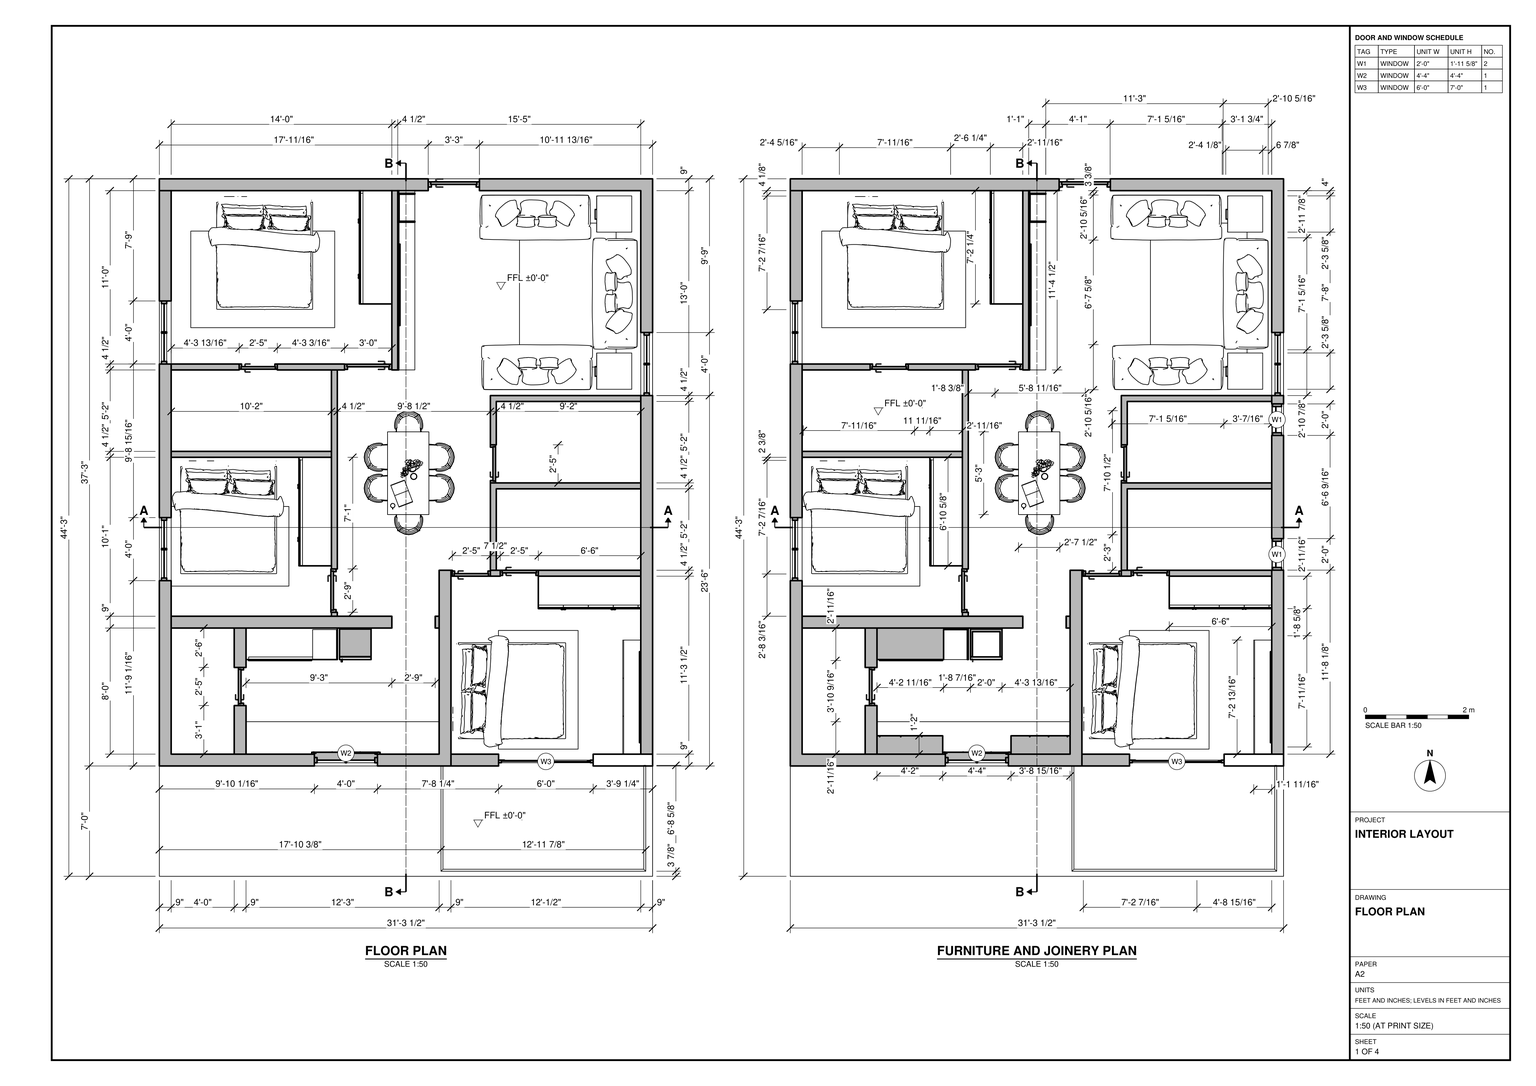
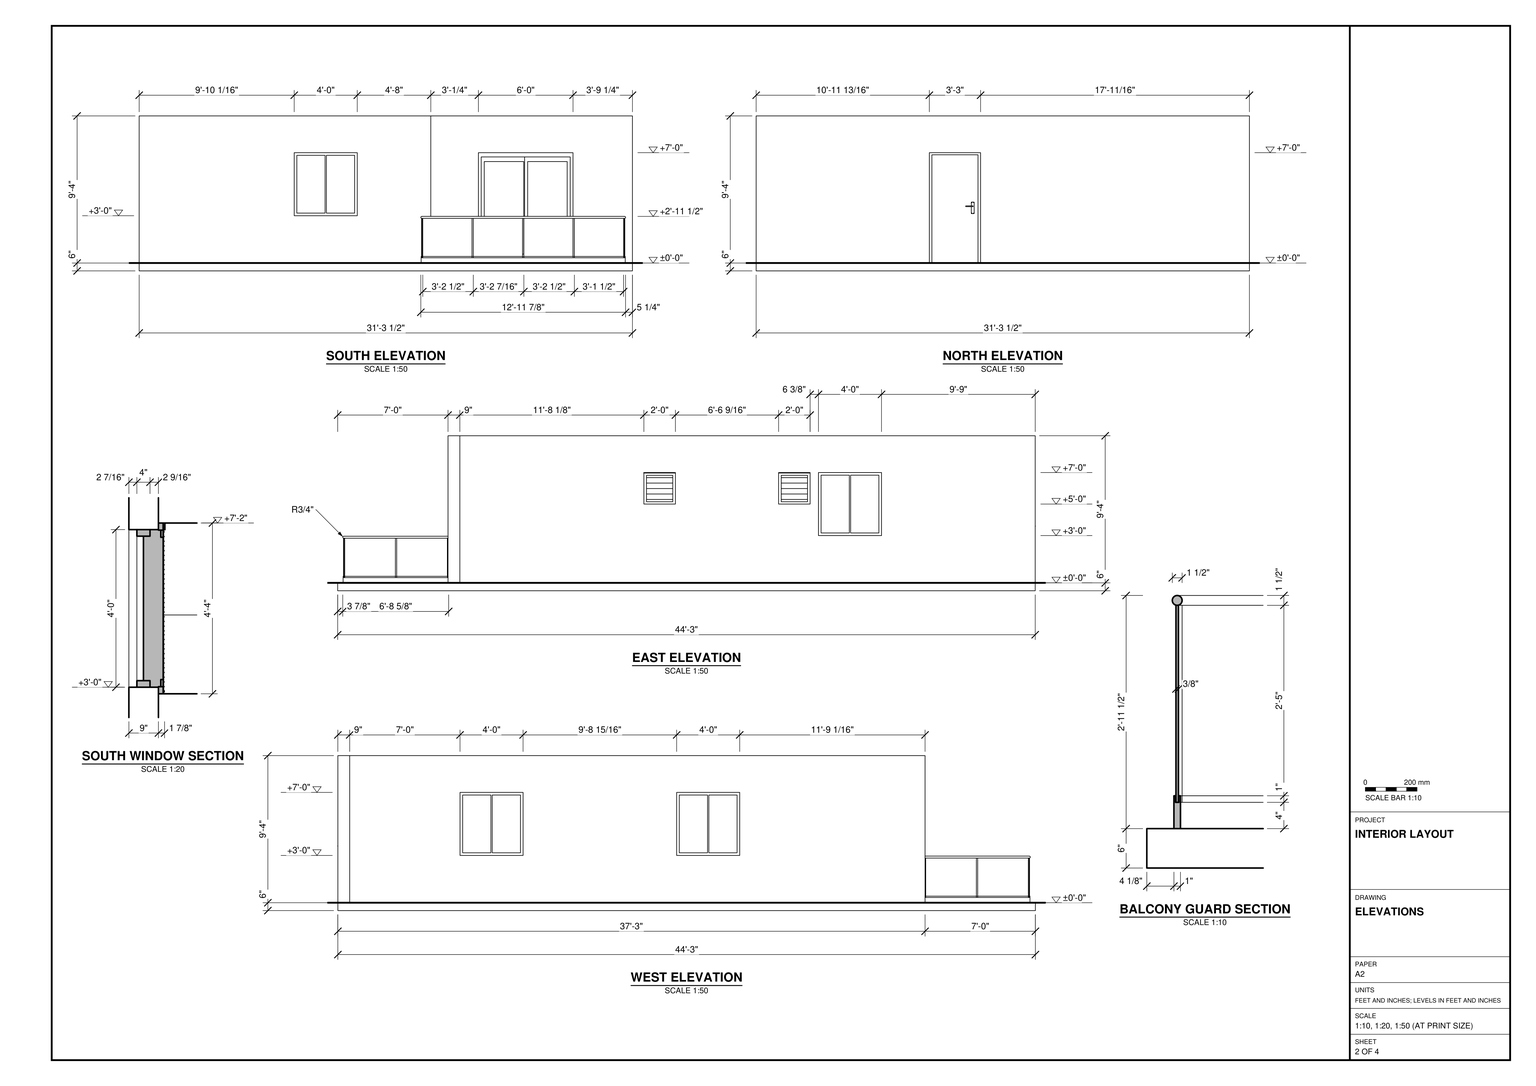
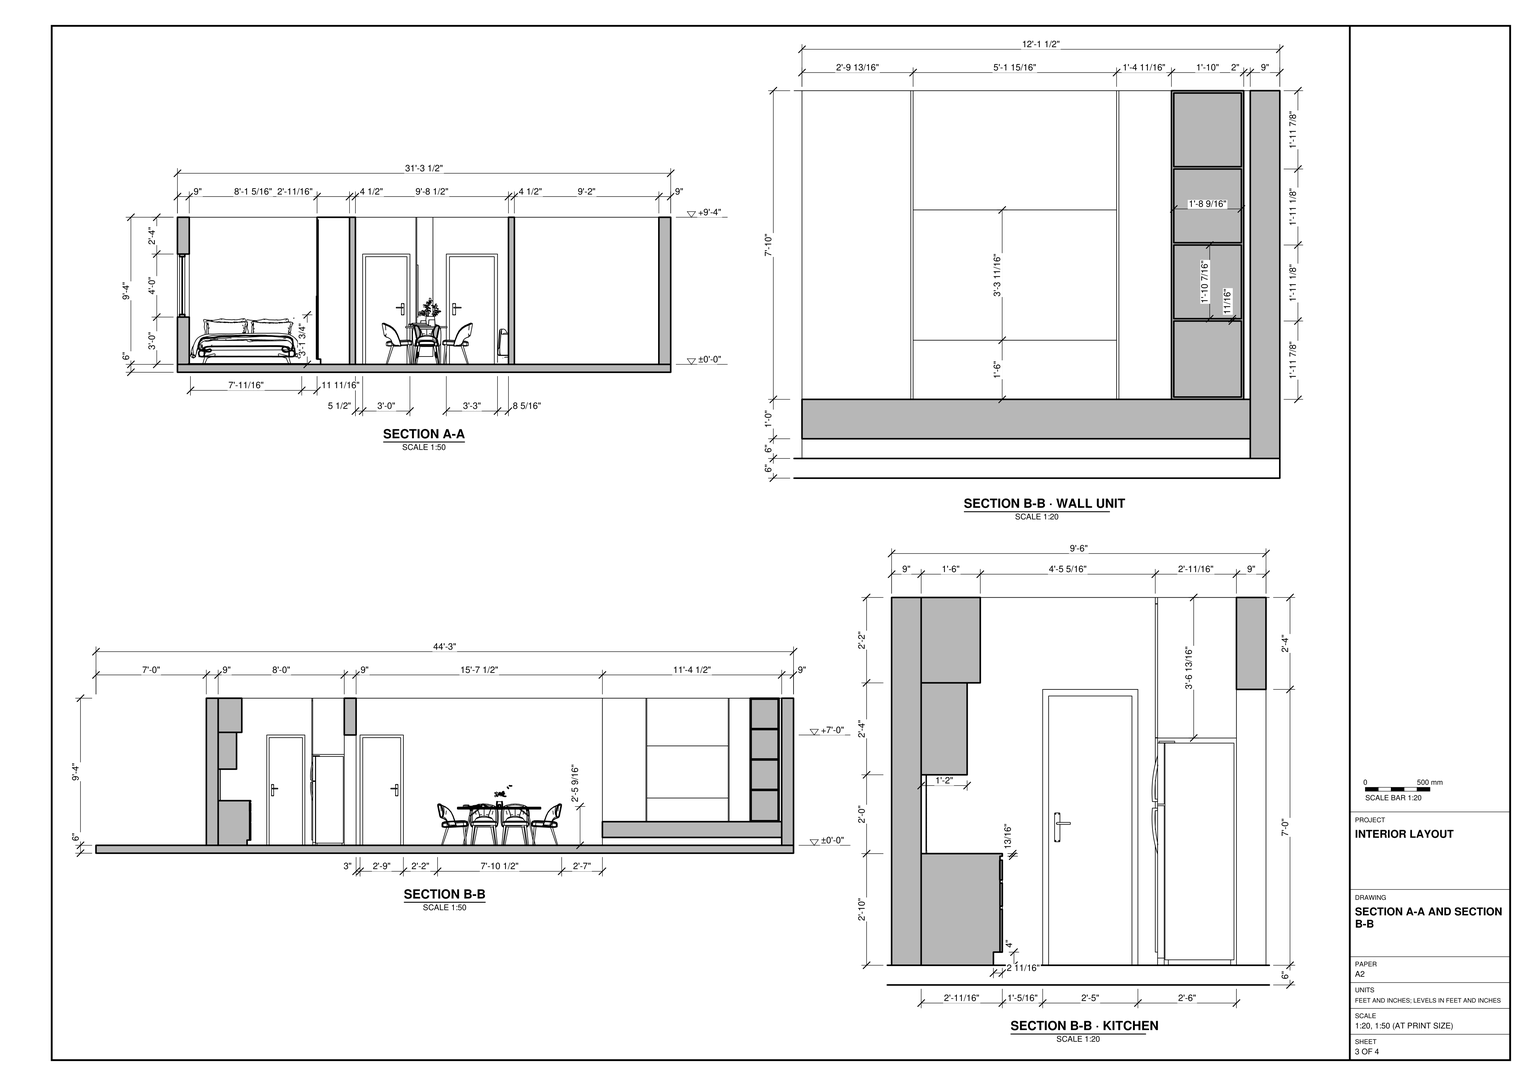
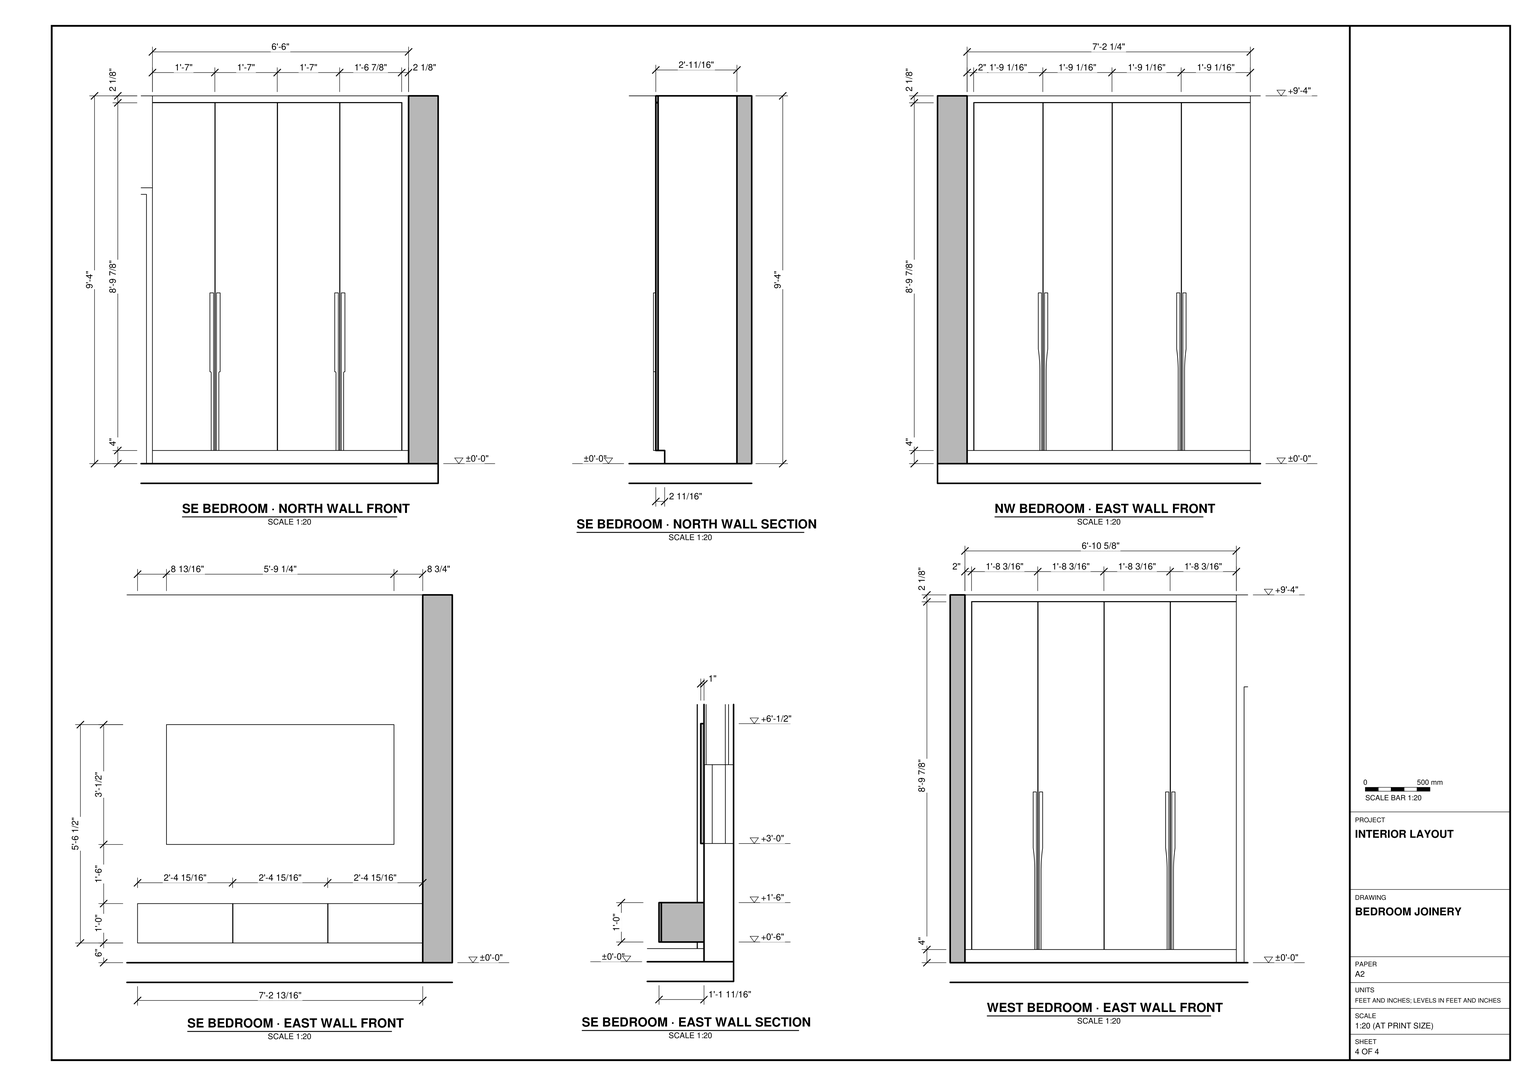
Build the single-storey interior in SketchUp using task_files/diagram_01.pdf. Work in feet and inches. Set the finished floor at ±0'-0". The overall model, including the balcony, is 31'-3 1/2" east to west, 44'-3 1/8" north to south and 9'-10" high.

Model the 6" floor slab and raise the walls 9'-4" above the finished floor. Follow the drawn wall thicknesses, distinguishing the 9" perimeter walls from the lighter 4 1/2" partitions. Lay out the bedrooms on the west side and at the southeast corner, the living area at the northeast, the central dining area and the kitchen at the southwest. Preserve the smaller enclosed rooms and the doorways connecting the spaces. Fit the doors, window units and high east-wall ventilators to the openings shown in plan and elevation. Extend the balcony outside the southeast bedroom and model its panelled glass guard using the guard section.

Use the furniture plan to size and orient the beds, bedroom storage, sofas, side tables, dining table and chairs. Use the sections to build the living-area wall unit with its low base and shelving, and the kitchen with its worktop, cabinets and refrigerator. Decor and loose items, including rugs, cushions and appliances, may be any suitable library components.

Keep the shell elements and each furniture or joinery piece in separate groups or components, and use components for repeated parts. Save one SketchUp model as output_files/furnished_three_bedroom_interior_with_a_south_balcony.skp.

# SketchUp Ruby script. Lengths in inches.
U = 1.inch
M = Sketchup.active_model
def pt(a) = Geom::Point3d.new(a.map { |v| v * U })
def face(e, loops, mat)
  f = e.add_face(loops[0].map { |a| pt(a) })
  loops[1..].each { |l| e.add_face(l.map { |a| pt(a) }).erase! }
  f.material = f.back_material = mat if mat
  f
end
# faces: each face lists its corners as indices into pts; further lists are holes
def faces(e, pts, list, mat = nil) = list.each { |f| face(e, (f[0].is_a?(Array) ? f : [f]).map { |l| l.map { |i| pts[i] } }, mat) }
# xy, xz, yz: faces in a plane at the given z, y or x. An outline is a flat list of corners, or four numbers for a rectangle; further outlines are holes
def ring(l) = l.size == 4 ? [[l[0], l[1]], [l[2], l[1]], [l[2], l[3]], [l[0], l[3]]] : l.each_slice(2).to_a
def flat(e, list, mat, &to3) = list.each { |f| face(e, (f[0].is_a?(Array) ? f : [f]).map { |l| ring(l).map { |u, v| to3.(u, v) } }, mat) }
def xy(e, z, list, mat = nil) = flat(e, list, mat) { |x, y| [x, y, z] }
def xz(e, y, list, mat = nil) = flat(e, list, mat) { |x, z| [x, y, z] }
def yz(e, x, list, mat = nil) = flat(e, list, mat) { |y, z| [x, y, z] }
def lines(e, pts, list) = list.each { |a, b| e.add_line(pt(pts[a]), pt(pts[b])) }
# prism: a flat outline (further loops are holes) pulled along v
def prism(e, loops, v, mat = nil)
  f = face(e, loops, mat); d = Geom::Vector3d.new(v.map { |x| x * U })
  f.pushpull(f.normal.samedirection?(d) ? d.length : -d.length)
end
def box(e, o, s, mat = nil) = prism(e, [[o, [o[0] + s[0], o[1], o[2]], [o[0] + s[0], o[1] + s[1], o[2]], [o[0], o[1] + s[1], o[2]]]], [0, 0, s[2]], mat)
def at(x, y, z, deg = 0) = Geom::Transformation.translation(pt([x, y, z])) * Geom::Transformation.rotation(ORIGIN, Z_AXIS, deg.degrees)
def axes(o, x, y, z) = Geom::Transformation.new([*x, 0, *y, 0, *z, 0, *pt(o).to_a, 1])
def part(name) = M.definitions.add(name)
# library, detail: a bought-in or finely detailed component or shape, given as its bounding box
def library(name, o, s) = part(name).tap { |d| box(d.entities, o, s) }
def detail(e, o, s) = box(e.add_group.entities, o, s)
def put(e, d, t, mat = nil) = e.add_instance(d, t).tap { |i| i.material = mat if mat }
def group(e, t, mat = nil) = e.add_group.tap { |g| g.transformation = t; g.material = mat if mat }.entities
root = M.entities
M.materials.add("0516 AP 9704 Lake Supreme-N").color = [0, 147, 150]
M.materials.add("0604 AP 9737 Aquamarine Pop-N").color = [0, 150, 118]
M.materials.add("0607 AP 9740 Bright Teal-N").color = [0, 121, 105]
M.materials.add("0908 AP 7841 CORN FIELD").color = [237, 222, 177]
M.materials.add("0916 AP 7849 PEBBLE MOSS").color = [210, 196, 159]
M.materials.add("0932 AP 7856 GOLDILOCKS").color = [236, 215, 152]
M.materials.add("0944 AP 9875 Lazy Daisy-N").color = [241, 200, 58]
M.materials.add("1160 AP 9961 Cherry Brown-N").color = [109, 68, 67]
M.materials.add("Carpet").color = [165, 157, 133]
M.materials.add("Railing Glass").color = [63, 150, 137]
M.materials["Railing Glass"].alpha = 0.13
M.materials.add("[Color M00]").color = [255, 255, 255]
M.materials.add("[Color M09]").color = [0, 0, 0]
M.materials.add("[Color_002]").color = [198, 198, 198]
M.materials.add("[Translucent Glass Gray]").color = [128, 128, 128]
M.materials["[Translucent Glass Gray]"].alpha = 0.5
M.materials.add("[Translucent Glass Tinted]1").color = [7, 201, 240]
M.materials["[Translucent Glass Tinted]1"].alpha = 0.48
M.materials.add("[Wood Cherry Original]").color = [152, 86, 42]
M.materials.add("[Wood Floor Parquet]").color = [145, 89, 39]
c1 = part("Sliding Window")
xy(c1.entities,0,[[0,0,66.93,1.97]],"[Color M09]")
xy(c1.entities,1.97,[[1.97,0,64.96,0,64.96,0.39,32.7,0.39,32.7,1.18,1.97,1.18],[34.23,1.18,64.96,1.97]],"[Color M09]")
xy(c1.entities,49.21,[[1.97,0,1.97,1.18,32.7,1.18,32.7,0.39,64.96,0.39,64.96,0],[34.23,1.18,64.96,1.97]],"[Color M09]")
xy(c1.entities,51.18,[[0,0,66.93,1.97]],"[Color M09]")
xz(c1.entities,0,[[[0,0,66.93,51.18],[1.97,1.97,64.96,49.21]]],"[Color M09]")
xz(c1.entities,1.18,[[[34.23,1.97,64.96,49.21],[34.85,4.12,62.81,47.07]]],"[Color M09]")
xz(c1.entities,1.97,[[[0,0,66.93,51.18],[1.97,1.97,64.96,49.21]]],"[Color M09]")
yz(c1.entities,0,[[0,0,1.97,51.18]],"[Color M09]")
yz(c1.entities,1.97,[[0,1.97,1.18,49.21]],"[Color M09]")
yz(c1.entities,64.96,[[0,1.97,0.39,49.21],[1.18,1.97,1.97,49.21]],"[Color M09]")
yz(c1.entities,66.93,[[0,0,1.97,51.18]],"[Color M09]")
g1 = group(c1.entities,at(1.97,0.39,1.97))
xy(g1,0,[[30.73,0,62.99,0.79],[0,0.79,32.26,1.57]])
xy(g1,2.15,[[32.88,0,60.84,0.79],[2.15,0.79,30.11,1.57]])
xy(g1,45.1,[[32.88,0,60.84,0.79],[2.15,0.79,30.11,1.57]],"[Translucent Glass Gray]")
xy(g1,47.24,[[30.73,0,62.99,0.79],[0,0.79,32.26,1.57]])
xz(g1,0,[[[30.73,0,62.99,47.24],[32.88,2.15,60.84,45.1]]])
xz(g1,0,[[32.88,2.15,60.84,45.1]],"[Translucent Glass Gray]")
xz(g1,0.79,[[[0,0,30.73,47.24],[2.15,2.15,30.11,45.1]],[30.73,0,32.26,47.24]])
xz(g1,0.79,[[2.15,2.15,30.11,45.1]],"[Translucent Glass Gray]")
xz(g1,1.57,[[[0,0,32.26,47.24],[2.15,2.15,30.11,45.1]]])
yz(g1,0,[[0.79,0,1.57,47.24]])
yz(g1,2.15,[[0.79,2.15,1.57,45.1]])
yz(g1,30.11,[[0.79,2.15,1.57,45.1]],"[Translucent Glass Gray]")
yz(g1,30.73,[[0,0,0.79,47.24]])
yz(g1,32.26,[[0.79,0,1.57,47.24]])
yz(g1,32.88,[[0,2.15,0.79,45.1]])
yz(g1,60.84,[[0,2.15,0.79,45.1]],"[Translucent Glass Gray]")
yz(g1,62.99,[[0,0,0.79,47.24]])
c2 = library("sofaD71839)",[0.35,-39.08,0.31],[80.46,34.29,30.24])
c3 = part("Drawer front")
xy(c3.entities,0,[[-0.39,0.08,15.35,0.63]])
xy(c3.entities,0.02,[[-0.375,0.63,15.34,0.71]])
xy(c3.entities,0.08,[[-0.31,0,15.28,0.08],[-0.31,0.08,15.28,0.71]])
xy(c3.entities,6.46,[[-0.31,0,15.28,0.08],[-0.31,0.08,15.28,0.71]])
xy(c3.entities,6.54,[[-0.39,0.08,15.35,0.63]])
xz(c3.entities,0,[[-0.31,0.08,15.28,6.46]])
xz(c3.entities,0.08,[[[-0.39,0,15.35,6.54],[-0.31,0.08,15.28,6.46]]])
xz(c3.entities,0.63,[[-0.39,0,-0.39,6.54,5.07,6.54,5.08,6.52,-0.375,6.52,-0.375,0.02,15.34,0.02,15.34,6.52,9.88,6.52,9.89,6.54,15.35,6.54,15.35,0]])
xz(c3.entities,0.71,[[[-0.375,0.02,15.34,6.52],[-0.31,0.08,15.28,6.46]]])
yz(c3.entities,-0.39,[[0.08,0,0.63,6.54]])
yz(c3.entities,-0.375,[[0.63,0.02,0.71,6.52]])
yz(c3.entities,-0.31,[[0,0.08,0.08,6.46],[0.08,0.08,0.71,6.46]])
yz(c3.entities,15.28,[[0,0.08,0.08,6.46],[0.08,0.08,0.71,6.46]])
yz(c3.entities,15.34,[[0.63,0.02,0.71,6.52]])
yz(c3.entities,15.35,[[0.08,0,0.63,6.54]])
p = [[10.63,0.08,5.23],[11.42,0.08,6.46],[9.06,0.08,5.23],[9.06,0,5.23]]
lines(c3.entities,p,[[0,1],[2,0],[2,3]])
c4 = part("Handle\#1")
xz(c4.entities,-32.1875,[[37.875,8.67,38.14,8.78,38.25,9.04,38.14,9.31,37.875,9.42,37.61,9.31,37.5,9.04,37.61,8.78]],"[Color_002]")
xz(c4.entities,-32.125,[[37.875,-2.58,38.14,-2.47,38.25,-2.21,38.14,-1.94,37.875,-1.83,37.61,-1.94,37.5,-2.21,37.61,-2.47]],"[Color_002]")
p = [[37.875,-32.125,-2.58],[37.61,-32.125,-2.47],[37.61,-29.86,-2.47],[37.875,-29.75,-2.58],[38.14,-32.125,-2.47],[38.14,-29.86,-2.47],
  [37.61,-29.86,9.31],[37.875,-29.75,9.42],[38.14,-29.86,9.31],[37.5,-32.125,-2.21],[37.5,-30.125,-2.21],[38.25,-32.125,-2.21],
  [38.25,-30.125,-2.21],[37.5,-30.125,9.04],[38.25,-30.125,9.04],[37.61,-32.125,-1.94],[37.61,-30.39,-1.94],[38.14,-32.125,-1.94],
  [38.14,-30.39,-1.94],[37.61,-30.39,8.78],[38.14,-30.39,8.78],[37.875,-32.125,-1.83],[37.875,-30.5,-1.83],[37.875,-30.5,8.67],
  [37.875,-32.1875,8.67],[37.61,-32.1875,8.78],[38.14,-32.1875,8.78],[37.5,-32.1875,9.04],[38.25,-32.1875,9.04],[37.61,-32.1875,9.31],
  [38.14,-32.1875,9.31],[37.875,-32.1875,9.42]]
faces(c4.entities,p,[[0,1,2,3],[4,0,3,5],[3,2,6,7],[5,3,7,8],[1,9,10,2],[11,4,5,12],[2,10,13,6],[12,5,8,14],
  [9,15,16,10],[17,11,12,18],[10,16,19,13],[18,12,14,20],[15,21,22,16],[21,17,18,22],[16,22,23,19],[22,18,20,23],
  [19,23,24,25],[23,20,26,24],[13,19,25,27],[20,14,28,26],[6,13,27,29],[14,8,30,28],[7,6,29,31],[8,7,31,30]],"[Color_002]")
c5 = part("Bedside cabinet")
put(c5.entities,c3,at(0.39,0,3.9375))
put(c5.entities,c3,at(0.39,0,10.47))
put(c5.entities,c4,axes([6.72,-12.04,-0.59],[0,0,0.3744],[0,-0.3744,0],[0.3744,0,0]))
put(c5.entities,c4,axes([6.72,-12.04,-6.875],[0,0,0.3744],[0,-0.3744,0],[0.3744,0,0]))
g2 = group(c5.entities,at(0,0,17.01))
box(g2,[0,0,0],[15.75,17.72,0.71])
g3 = group(c5.entities,at(15.35,0,16.14))
box(g3,[0,0.71,-12.2],[0.39,17.01,13.07])
g4 = group(c5.entities,at(0,0,16.14))
box(g4,[0,0.71,-12.2],[0.39,17.01,13.07])
g5 = group(c5.entities,at(0,0,0))
box(g5,[0,0,0],[15.75,17.72,3.9375])
g6 = group(c5.entities,at(18.11,17.32,16.14))
box(g6,[-17.72,0,-12.2],[14.96,0.39,13.07])
c6 = library("Спалня Венид",[0.07,-0.07,0],[84.71,86.8,39])
c7 = part("Tapete")
box(c7.entities,[0,0,0],[73.55,109.57,0.42],"Carpet")
c8 = part("02 Tapete")
put(c8.entities,c7,at(0.05,-109.34,0))
c9 = part("Carpet")
put(c9.entities,c8,at(0,0,0))
c10 = part("ventilator\#1")
g7 = group(c10.entities,at(0,0,0))
xy(g7,0,[[0,0,24,1],[0,1,24,6.83]],"[Wood Floor Parquet]")
xy(g7,1.75,[[2,0,22,6.83]],"[Wood Floor Parquet]")
xy(g7,21.87,[[2,0,22,6.83]],"[Wood Cherry Original]")
xy(g7,23.62,[[0,0,24,1],[0,1,24,6.83]],"[Wood Floor Parquet]")
xz(g7,0,[[[0,0,24,23.62],[2,1.75,22,21.87]]],"[Wood Floor Parquet]")
xz(g7,6.83,[[[0,0,24,23.62],[2,1.75,22,21.87]]],"[Wood Cherry Original]")
yz(g7,0,[[0,0,1,23.62],[1,0,6.83,23.62]],"[Wood Floor Parquet]")
yz(g7,2,[[0,1.75,6.83,1.75,6.83,7.66,0,3.5],[0,3.5,6.83,7.66,6.83,11.8125,0,7.66],[0,7.66,6.83,11.8125,6.83,15.97,0,11.8125],[0,11.8125,6.83,15.97,6.83,20.12,0,15.97],[0,15.97,6.83,20.12,6.83,21.87,0,21.87]],"[Wood Floor Parquet]")
yz(g7,22,[[0,1.75,0,3.5,6.83,7.66,6.83,1.75],[0,3.5,0,7.66,6.83,11.8125,6.83,7.66],[0,7.66,0,11.8125,6.83,15.97,6.83,11.8125],[0,11.8125,0,15.97,6.83,20.12,6.83,15.97],[0,15.97,0,21.87,6.83,21.87,6.83,20.12]],"[Wood Floor Parquet]")
yz(g7,24,[[0,0,1,23.62],[1,0,6.83,23.62]],"[Wood Floor Parquet]")
p = [[2,0,3.5],[2,6.83,7.66],[22,6.83,7.66],[22,0,3.5],[2,6.83,11.8125],[2,0,7.66],
  [22,0,7.66],[22,6.83,11.8125],[2,0,11.8125],[2,6.83,15.97],[22,6.83,15.97],[22,0,11.8125],
  [2,6.83,20.12],[2,0,15.97],[22,0,15.97],[22,6.83,20.12]]
faces(g7,p,[[0,1,2,3],[4,5,6,7],[8,9,10,11]],"[Translucent Glass Tinted]1")
faces(g7,p,[[12,13,14,15]],"[Translucent Glass Gray]")
c11 = library("Refridgerator",[117.47,47.52,0],[24,24.96,68.0625])
c12 = library("DINING SET",[25.27,8.07,0],[68.7,94.48,53.71])
c13 = library("Window with blinds",[0,0,0],[5.61,36,36])
c14 = part("Group15\#1")
xy(c14.entities,0,[[0,84,0,522,9,522,9,93,213,93,213,233,222,233,222,84]])
xy(c14.entities,36,[[118.03,84,166.03,93],[0,225.09,9,273.09],[0,390,9,438]])
xy(c14.entities,84,[[118.03,84,166.03,93],[0,225.09,9,273.09],[0,390,9,438]])
xy(c14.entities,112,[[0,84,222,84,222,233,213,233,213,93,9,93,9,522,0,522]])
xz(c14.entities,84,[[[0,0,222,112],[118.03,36,166.03,84]]])
xz(c14.entities,93,[[[9,0,213,112],[118.03,36,166.03,84]]])
xz(c14.entities,225.09,[[0,36,9,84]])
xz(c14.entities,233,[[213,0,222,112]])
xz(c14.entities,273.09,[[0,36,9,84]])
xz(c14.entities,390,[[0,36,9,84]])
xz(c14.entities,438,[[0,36,9,84]])
xz(c14.entities,522,[[0,0,9,112]])
yz(c14.entities,0,[[[84,0,522,112],[225.09,36,273.09,84],[390,36,438,84]]])
yz(c14.entities,9,[[[93,0,522,112],[225.09,36,273.09,84],[390,36,438,84]]])
yz(c14.entities,118.03,[[84,36,93,84]])
yz(c14.entities,166.03,[[84,36,93,84]])
yz(c14.entities,213,[[93,0,233,112]])
yz(c14.entities,222,[[84,0,233,112]])
c15 = part("Group17\#1")
xy(c15.entities,0,[[366.5,93,366.5,522,243.66,522,243.66,531,375.5,531,375.5,93],[0,522,204.66,531]])
xy(c15.entities,36,[[366.5,366,375.5,414]])
xy(c15.entities,60,[[366.5,233.11,375.5,257.11],[366.5,335.65,375.5,359.65]])
xy(c15.entities,84,[[366.5,233.11,375.5,257.11],[366.5,335.65,375.5,359.65],[366.5,366,375.5,414],[204.66,522,243.66,531]])
xy(c15.entities,112,[[366.5,93,375.5,93,375.5,531,0,531,0,522,366.5,522]])
xz(c15.entities,93,[[366.5,0,375.5,112]])
xz(c15.entities,233.11,[[366.5,60,375.5,84]])
xz(c15.entities,257.11,[[366.5,60,375.5,84]])
xz(c15.entities,335.65,[[366.5,60,375.5,84]])
xz(c15.entities,359.65,[[366.5,60,375.5,84]])
xz(c15.entities,366,[[366.5,36,375.5,84]])
xz(c15.entities,414,[[366.5,36,375.5,84]])
xz(c15.entities,522,[[0,0,204.66,0,204.66,84,243.66,84,243.66,0,366.5,0,366.5,112,0,112]])
xz(c15.entities,531,[[0,0,0,112,375.5,112,375.5,0,243.66,0,243.66,84,204.66,84,204.66,0]])
yz(c15.entities,0,[[522,0,531,112]])
yz(c15.entities,204.66,[[522,0,531,84]])
yz(c15.entities,243.66,[[522,0,531,84]])
yz(c15.entities,366.5,[[[93,0,522,112],[366,36,414,84],[335.65,60,359.65,84],[233.11,60,257.11,84]]])
yz(c15.entities,375.5,[[[93,0,531,112],[366,36,414,84],[335.65,60,359.65,84],[233.11,60,257.11,84]]])
c16 = part("Group18\#1")
prism(c16.entities,[[[213,198,0],[210,198,0],[210,198,84],[177,198,84],[177,198,0],[9,198,0],[9,198,112],[213,198,112]]],[0,-9,0])
c17 = part("Group19\#1")
prism(c17.entities,[[[66,93,0],[66,130,0],[66,130,84],[66,159,84],[66,159,0],[66,189,0],[66,189,112],[66,93,112]]],[-9,0,0])
c18 = part("Group21\#1")
xy(c18.entities,0,[[9,385.5,60.78,390],[89.78,385.5,141,390],[177,385.5,181.5,522],[181.5,385.5,182.21,522]])
xy(c18.entities,18,[[181.5,418.625,182.21,419.33],[181.5,481.29,182.21,482]])
xy(c18.entities,84,[[60.78,385.5,89.78,390],[141,385.5,177,390]])
xy(c18.entities,112,[[9,385.5,181.5,385.5,181.5,522,177,522,177,390,9,390],[181.5,418.625,182.21,419.33],[181.5,481.29,182.21,482],[181.5,482,182.21,522]])
xy(c18.entities,112,[[181.5,385.5,182.21,418.625],[181.5,419.33,182.21,481.29]],"0916 AP 7849 PEBBLE MOSS")
xz(c18.entities,385.5,[[9,0,60.78,0,60.78,84,89.78,84,89.78,0,141,0,141,84,177,84,177,0,181.5,0,181.5,112,9,112]])
xz(c18.entities,385.5,[[181.5,0,182.21,112]],"0916 AP 7849 PEBBLE MOSS")
xz(c18.entities,390,[[9,0,9,112,177,112,177,84,141,84,141,0,89.78,0,89.78,84,60.78,84,60.78,0]])
xz(c18.entities,418.625,[[181.5,18,182.21,112]])
xz(c18.entities,419.33,[[181.5,18,182.21,112]])
xz(c18.entities,481.29,[[181.5,18,182.21,112]])
xz(c18.entities,482,[[181.5,18,182.21,112]])
xz(c18.entities,522,[[177,0,181.5,112],[181.5,0,182.21,112]])
yz(c18.entities,9,[[385.5,0,390,112]])
yz(c18.entities,60.78,[[385.5,0,390,84]])
yz(c18.entities,89.78,[[385.5,0,390,84]])
yz(c18.entities,141,[[385.5,0,390,84]])
yz(c18.entities,177,[[385.5,0,390,84],[390,0,522,112]])
yz(c18.entities,181.5,[[385.5,0,385.5,112,418.625,112,418.625,18,419.33,18,419.33,112,481.29,112,481.29,18,482,18,482,112,522,112,522,0],[418.625,18,419.33,112],[481.29,18,482,112]])
yz(c18.entities,182.21,[[385.5,0,522,0,522,112,482,112,482,18,481.29,18,481.29,112,419.33,112,419.33,18,418.625,18,418.625,112,385.5,112]],"0916 AP 7849 PEBBLE MOSS")
yz(c18.entities,182.21,[[418.625,18,419.33,112],[481.29,18,482,112]],"0944 AP 9875 Lazy Daisy-N")
c19 = part("Group22\#1")
prism(c19.entities,[[[135.5,198,0],[135.5,201,0],[135.5,201,84],[135.5,234,84],[135.5,234,0],[135.5,385.5,0],[135.5,385.5,112],[135.5,198,112]]],[-4.5,0,0])
c20 = part("Group23\#1")
box(c20.entities,[9,319,0],[122,4.5,112])
c21 = part("Group24\#1")
xy(c21.entities,0,[[252,328.5,252,366,366.5,366,366.5,361.5,256.5,361.5,256.5,328.5]])
xy(c21.entities,84,[[252,299.5,256.5,328.5]])
xy(c21.entities,112,[[252,299.5,256.5,299.5,256.5,361.5,366.5,361.5,366.5,366,252,366]])
xz(c21.entities,299.5,[[252,84,256.5,112]])
xz(c21.entities,328.5,[[252,0,256.5,84]])
xz(c21.entities,361.5,[[256.5,0,366.5,112]])
xz(c21.entities,366,[[252,0,366.5,112]])
yz(c21.entities,252,[[328.5,0,328.5,84,299.5,84,299.5,112,366,112,366,0]])
yz(c21.entities,256.5,[[328.5,0,361.5,0,361.5,112,299.5,112,299.5,84,328.5,84]])
yz(c21.entities,366.5,[[361.5,0,366,112]])
c22 = part("Group25\#1")
prism(c22.entities,[[[252,228.5,0],[259.5,228.5,0],[259.5,228.5,84],[288.5,228.5,84],[288.5,228.5,0],[366.5,228.5,0],[366.5,228.5,112],[222,228.5,112],[222,228.5,0],[223,228.5,0],[223,228.5,84],[252,228.5,84]]],[0,4.5,0])
c23 = part("Group26\#1")
prism(c23.entities,[[[366.5,295,0],[256.5,295,0],[256.5,233,0],[252,233,0],[252,299.5,0],[366.5,299.5,0]]],[0,0,112])
c24 = part("Group26\#2")
prism(c24.entities,[[[375.5,93,0],[330.25,93,0],[330.25,93,84],[258.25,93,84],[258.25,93,0],[222,93,0],[222,93,112],[375.5,93,112]]],[0,-9,0])
c25 = library("Glass Railing",[-0.75,-80.125,0],[155.875,80.625,35.5])
c26 = part("Group46\#3")
xy(c26.entities,0,[[-22,-22,-0.5,22],[0.5,-22,22,22]])
c27 = part("Group45\#5")
prism(c27.entities,[[[-24,24,0],[24,24,0],[24,-24,0],[-24,-24,0]],[[0.5,22,0],[0.5,-22,0],[22,-22,0],[22,22,0]],[[-22,-22,0],[-0.5,-22,0],[-0.5,22,0],[-22,22,0]]],[0,0,4])
put(c27.entities,c26,at(0,0,2),"[Translucent Glass Gray]")
c28 = part("Group45\#4")
prism(c28.entities,[[[-24,24,0],[24,24,0],[24,-24,0],[-24,-24,0]],[[0.5,22,0],[0.5,-22,0],[22,-22,0],[22,22,0]],[[-22,-22,0],[-0.5,-22,0],[-0.5,22,0],[-22,22,0]]],[0,0,4])
put(c28.entities,c26,at(0,0,2),"[Translucent Glass Gray]")
c29 = part("Group45\#3")
prism(c29.entities,[[[-24,24,0],[24,24,0],[24,-24,0],[-24,-24,0]],[[0.5,22,0],[0.5,-22,0],[22,-22,0],[22,22,0]],[[-22,-22,0],[-0.5,-22,0],[-0.5,22,0],[-22,22,0]]],[0,0,4])
put(c29.entities,c26,at(0,0,2),"[Translucent Glass Gray]")
c30 = part("Group45\#1")
prism(c30.entities,[[[-24,24,0],[24,24,0],[24,-24,0],[-24,-24,0]],[[0.5,22,0],[0.5,-22,0],[22,-22,0],[22,22,0]],[[-22,-22,0],[-0.5,-22,0],[-0.5,22,0],[-22,22,0]]],[0,0,4])
put(c30.entities,c26,at(0,0,2),"[Translucent Glass Gray]")
c31 = library("Group\#18",[0,0,0],[31.5,6.69,82.68])
c32 = library("Group\#19",[0,0,0],[31.5,6.69,82.68])
c33 = library("Group\#20",[0,0,0],[31.5,6.69,82.68])
c34 = part("Group\#32")
xy(c34.entities,0,[[0.39,-0.71,1.1,0]],"[Color M09]")
xy(c34.entities,48,[[0,-0.71,1.1,0]],"[Color M09]")
xz(c34.entities,-0.71,[[0.39,0,1.1,0,1.1,48,0,48,0,24,0.12,23.99,0.22,23.96,0.3,23.9,0.35,23.82,0.38,23.72,0.39,23.6]],"[Color M09]")
xz(c34.entities,0,[[0.39,0,0.39,23.6,0.38,23.72,0.35,23.82,0.3,23.9,0.22,23.96,0.12,23.99,0,24,0,48,1.1,48,1.1,0]])
yz(c34.entities,0,[[-0.71,24,0,48]],"[Color M09]")
yz(c34.entities,0.39,[[-0.71,0,0,23.6]],"[Color M09]")
yz(c34.entities,1.1,[[-0.71,0,0,48]],"[Color M09]")
p = [[0.38,-0.71,23.72],[0.38,0,23.72],[0.39,0,23.6],[0.39,-0.71,23.6],[0.35,-0.71,23.82],[0.35,0,23.82],
  [0.3,-0.71,23.9],[0.3,0,23.9],[0.22,-0.71,23.96],[0.22,0,23.96],[0,-0.71,24],[0,0,24],
  [0.12,0,23.99],[0.12,-0.71,23.99]]
faces(c34.entities,p,[[0,1,2,3],[4,5,1,0],[6,7,5,4],[8,9,7,6],[10,11,12,13],[13,12,9,8]],"[Color M09]")
c35 = part("Group\#35")
prism(c35.entities,[[[0,0.71,0],[0,0.71,48],[1.1,0.71,48],[1.1,0.71,24],[0.98,0.71,23.99],[0.88,0.71,23.96],[0.81,0.71,23.9],[0.75,0.71,23.83],[0.72,0.71,23.73],[0.71,0.71,23.61],[0.71,0.71,0]]],[0,-0.71,0])
c36 = part("Group\#36")
prism(c36.entities,[[[0.71,0.51,24],[0.71,0.51,24.58],[0.71,0.52,25.16],[0.71,0.54,25.74],[0.71,0.56,26.31],[0.71,0.59,26.89],[0.71,0.625,27.47],[0.71,0.67,28.05],[0.71,0.72,28.625],[0.71,0.77,29.2],[0.71,0.84,29.78],[0.71,0.91,30.35],[0.71,0.98,30.92],[0.71,0.98,48],[0.71,0,48],[0.71,0,0],[0.71,0.51,0]]],[-0.71,0,0])
c37 = library("Group\#48",[0,0,0],[147,24.71,34])
put(root,c1,axes([258.25,86.5,0],[1.07576,0,0],[0,1,0],[0,0,1.64123]))
put(root,c2,axes([368.61,486.51,0],[0,-1.06,0],[1,0,0],[0,0,1]))
put(root,c2,axes([330.45,365.66,-0.31],[-1.06,0,0],[0,-1,0],[0,0,1]))
put(root,c2,axes([329.14,523.43,-0.31],[-1.06,0,0],[0,1,0],[0,0,1]))
put(root,c5,axes([332.89,398.39,0],[0,-1.7538,0],[1.5096,0,0],[0,0,1.11]))
put(root,c5,axes([332.89,518.02,0],[0,-1.7538,0],[1.5096,0,0],[0,0,1.11]))
put(root,c6,at(37.26,431.48,0))
put(root,c6,at(9.84,230.24,-0.55))
put(root,c9,at(274.12,497.04,0))
put(root,c9,at(24.17,417.62,0,90))
put(root,c9,axes([8.49,220.88,0],[0,0.8245,0],[-0.8245,0,0],[0,0,0.8245]))
put(root,c10,at(373.98,233.11,60,90))
put(root,c10,at(373.98,335.65,60,90))
put(root,c11,at(19.71,115.77,0.16))
put(root,c12,at(130.59,251.94,0))
put(root,c9,axes([318.83,97.03,0.59],[-0.8245,0,0],[0,-0.8245,0],[0,0,0.8245]))
put(root,c6,at(309.47,98.38,0.04,90))
put(root,c13,axes([116.03,94.96,34],[0,-0.35,0],[1.44444,0,0],[0,0,1.44444]))
put(root,c14,at(0,0,0))
put(root,c15,at(0,0,0))
put(root,c16,at(0,0,0))
put(root,c17,at(0,0,0))
put(root,c18,at(0,0,0))
put(root,c19,at(0,0,0))
put(root,c20,at(0,0,0))
put(root,c21,at(0,0,0))
g8 = group(root,at(0,0,-6))
box(g8,[0,0,0],[375.5,531,6])
put(root,c22,at(0,0,0))
put(root,c23,at(0,0,0))
put(root,c24,at(0,0,0))
put(root,c25,at(215.15,84,0))
g9 = group(root,at(369,366,36))
p = [[0,0,48],[0,0,0],[0,48,0],[0,48,48]]
lines(g9,p,[[0,1],[1,2],[2,3],[3,0]])
put(g9,c27,axes([0,24,24],[0,1,0],[0,0,1],[1,0,0]),"[Color M09]")
g10 = group(root,at(1.61,390,36))
p = [[0,0,48],[0,0,0],[0,48,0],[0,48,48]]
lines(g10,p,[[0,1],[1,2],[2,3],[3,0]])
put(g10,c28,axes([0,24,24],[0,1,0],[0,0,1],[1,0,0]),"[Color M09]")
g11 = group(root,at(1.61,225.09,36))
p = [[0,0,48],[0,0,0],[0,48,0],[0,48,48]]
lines(g11,p,[[0,1],[1,2],[2,3],[3,0]])
put(g11,c29,axes([0,24,24],[0,1,0],[0,0,1],[1,0,0]),"[Color M09]")
g12 = group(root,at(118.03,90.4375,36,-90),"Railing Glass")
p = [[0,0,48],[0,0,0],[0,48,0],[0,48,48]]
lines(g12,p,[[0,1],[1,2],[2,3],[3,0]])
put(g12,c30,axes([0,24,24],[0,1,0],[0,0,1],[1,0,0]),"[Color M09]")
put(root,c31,axes([204.66,524.45,0],[1.23825,0,0],[0,1,0],[0,0,1.016]))
put(root,c32,axes([223,232.75,0],[0.92075,0,0],[0,-1,0],[0,0,1.016]))
put(root,c32,axes([134.84,234,0],[0,-1.04775,0],[-1,0,0],[0,0,1.016]))
put(root,c32,axes([177,385.62,0],[-1.143,0,0],[0,1,0],[0,0,1.016]))
put(root,c33,axes([60.78,390.31,0],[0.92075,0,0],[0,-1,0],[0,0,1.016]))
put(root,c33,axes([251.69,299.5,0],[0,0.92075,0],[1,0,0],[0,0,1.016]))
put(root,c33,axes([64.4375,130,0],[0,0.92075,0],[-1,0,0],[0,0,1.016]))
put(root,c33,axes([259.5,228.75,0],[0.92075,0,0],[0,1,0],[0,0,1.016]))
g13 = group(root,at(288.5,204.5,0),"0516 AP 9704 Lake Supreme-N")
xy(g13,0,[[0,2,78,24]])
xy(g13,4,[[0,-0.71,19,0],[19.12,-0.71,38,0],[38.12,-0.71,57,0],[57.12,-0.71,75.88,0],[76,-0.71,78,0],
  [0,0,19,2],[19,0,19.12,2],[19.12,0,38,2],[38,0,38.12,2],[38.12,0,57,2],
  [57,0,57.12,2],[57.12,0,75.88,2],[75.88,0,76,2],[76,0,78,2]])
xy(g13,109.88,[[0,-0.71,19,0],[19.12,-0.71,38,0],[38.12,-0.71,57,0],[57.12,-0.71,75.88,0]])
xy(g13,110,[[0,-0.71,76,0]])
xy(g13,112,[[0,-0.71,78,0]])
xy(g13,112,[[0,0,78,24]],"[Color M00]")
xz(g13,-0.71,[[0,4,19,109.88],[76,4,78,4,78,112,0,112,0,110,76,110],[19.12,4,38,109.88],[38.12,4,57,109.88],[57.12,4,75.88,109.88]])
xz(g13,0,[[0,4,19,109.88],[19,4,19.12,4,19.12,109.88,38,109.88,38,4,38.12,4,38.12,109.88,57,109.88,57,4,57.12,4,57.12,109.88,75.88,109.88,75.88,4,76,4,76,110,0,110,0,109.88,19,109.88],[76,4,76,110,0,110,0,112,78,112,78,4],[19.12,4,38,109.88],[38.12,4,57,109.88],
  [57.12,4,75.88,109.88]])
xz(g13,2,[[0,0,78,4]])
xz(g13,24,[[0,0,78,112]])
yz(g13,0,[[-0.71,4,0,109.88],[-0.71,110,0,112]])
yz(g13,0,[[2,0,2,4,0,4,0,112,24,112,24,0]],"[Color M00]")
yz(g13,19,[[-0.71,4,0,109.88]])
yz(g13,19.12,[[-0.71,4,0,109.88]])
yz(g13,38,[[-0.71,4,0,109.88]])
yz(g13,38.12,[[-0.71,4,0,109.88]])
yz(g13,57,[[-0.71,4,0,109.88]])
yz(g13,57.12,[[-0.71,4,0,109.88]])
yz(g13,75.88,[[-0.71,4,0,109.88]])
yz(g13,76,[[-0.71,4,0,110]])
yz(g13,78,[[2,0,24,0,24,112,0,112,0,4,2,4],[-0.71,4,0,112]])
g14 = group(root,at(107,236.37,0),"0607 AP 9740 Bright Teal-N")
xy(g14,0,[[2,0,24,82.63]])
xy(g14,4,[[-0.71,0,0,20.04],[0,0,2,80.63],[-0.71,20.16,0,40.2],[-0.71,40.32,0,60.36],[-0.71,60.47,0,80.51],
  [-0.71,80.63,2,82.63]])
xy(g14,109.88,[[-0.71,0,0,20.04],[-0.71,20.16,0,40.2],[-0.71,40.32,0,60.36],[-0.71,60.47,0,80.51]])
xy(g14,110,[[-0.71,0,0,40.2],[-0.71,40.2,0,40.32],[-0.71,40.32,0,80.63]])
xy(g14,112,[[-0.71,0,24,82.63]],"[Color M00]")
xz(g14,0,[[-0.71,4,0,109.88]])
xz(g14,0,[[2,0,24,0,24,112,-0.71,112,-0.71,110,0,110,0,4,2,4]],"[Color M00]")
xz(g14,20.04,[[-0.71,4,0,109.88]])
xz(g14,20.16,[[-0.71,4,0,109.88]])
xz(g14,40.2,[[-0.71,4,0,109.88]])
xz(g14,40.32,[[-0.71,4,0,109.88]])
xz(g14,60.36,[[-0.71,4,0,109.88]])
xz(g14,60.47,[[-0.71,4,0,109.88]])
xz(g14,80.51,[[-0.71,4,0,109.88]])
xz(g14,80.63,[[-0.71,4,0,110]])
xz(g14,82.63,[[2,0,2,4,-0.71,4,-0.71,112,24,112,24,0]])
yz(g14,-0.71,[[0,4,20.04,109.88],[80.63,4,80.63,110,0,110,0,112,82.63,112,82.63,4],[20.16,4,40.2,109.88],[40.32,4,60.36,109.88],[60.47,4,80.51,109.88]])
yz(g14,0,[[0,4,20.04,109.88],[20.04,4,20.04,109.88,0,109.88,0,110,40.2,110,40.2,109.88,20.16,109.88,20.16,4],[20.16,4,40.2,109.88],[40.2,4,40.32,110],[40.32,4,60.36,109.88],
  [60.36,4,60.36,109.88,40.32,109.88,40.32,110,80.63,110,80.63,4,80.51,4,80.51,109.88,60.47,109.88,60.47,4],[60.47,4,80.51,109.88]])
yz(g14,2,[[0,0,82.63,4]])
yz(g14,24,[[0,0,82.63,112]])
g15 = group(root,at(153,435.74,0),"1160 AP 9961 Cherry Brown-N")
xy(g15,0,[[2,0,24,86.26]])
xy(g15,4,[[-0.71,0,0,20.95],[0,0,2,84.26],[-0.71,21.0625,0,42.01],[-0.71,42.13,0,63.07],[-0.71,63.19,0,84.14],
  [-0.71,84.26,0,86.26],[0,84.26,2,86.26]])
xy(g15,109.88,[[-0.71,0,0,20.95],[-0.71,21.0625,0,42.01],[-0.71,42.13,0,63.07],[-0.71,63.19,0,84.14]])
xy(g15,110,[[-0.71,0,0,84.26]])
xy(g15,112,[[-0.71,0,0,86.26]])
xy(g15,112,[[0,0,24,86.26]],"[Color M00]")
xz(g15,0,[[-0.71,4,0,109.88],[-0.71,110,0,112]])
xz(g15,0,[[2,0,24,0,24,112,0,112,0,4,2,4]],"[Color M00]")
xz(g15,20.95,[[-0.71,4,0,109.88]])
xz(g15,21.0625,[[-0.71,4,0,109.88]])
xz(g15,42.01,[[-0.71,4,0,109.88]])
xz(g15,42.13,[[-0.71,4,0,109.88]])
xz(g15,63.07,[[-0.71,4,0,109.88]])
xz(g15,63.19,[[-0.71,4,0,109.88]])
xz(g15,84.14,[[-0.71,4,0,109.88]])
xz(g15,84.26,[[-0.71,4,0,110]])
xz(g15,86.26,[[2,0,2,4,0,4,0,112,24,112,24,0],[-0.71,4,0,112]])
yz(g15,-0.71,[[0,4,20.95,109.88],[84.26,4,84.26,110,0,110,0,112,86.26,112,86.26,4],[21.0625,4,42.01,109.88],[42.13,4,63.07,109.88],[63.19,4,84.14,109.88]])
yz(g15,0,[[0,4,20.95,109.88],[20.95,4,20.95,109.88,0,109.88,0,110,84.26,110,84.26,4,84.14,4,84.14,109.88,63.19,109.88,63.19,4,63.07,4,63.07,109.88,42.13,109.88,42.13,4,42.01,4,42.01,109.88,21.0625,109.88,21.0625,4],[84.26,4,86.26,4,86.26,112,0,112,0,110,84.26,110],[21.0625,4,42.01,109.88],[42.13,4,63.07,109.88],
  [63.19,4,84.14,109.88]])
yz(g15,2,[[0,0,86.26,4]])
yz(g15,24,[[0,0,86.26,112]])
put(root,c34,at(306,203.79,4))
put(root,c35,at(308.01,203.08,4),"[Color M09]")
put(root,c34,at(344,203.79,4))
put(root,c35,at(346.01,203.08,4),"[Color M09]")
put(root,c36,at(105.58,297.24,4),"[Color M09]")
put(root,c36,axes([105.58,296.33,4],[1,0,0],[0,-1,0],[0,0,1]),"[Color M09]")
put(root,c36,axes([105.58,256.01,4],[1,0,0],[0,-1,0],[0,0,1]),"[Color M09]")
put(root,c36,at(105.58,256.92,4),"[Color M09]")
put(root,c36,axes([151.58,498.42,4],[1,0,0],[0,-1,0],[0,0,1]),"[Color M09]")
put(root,c36,at(151.58,499.33,4),"[Color M09]")
put(root,c36,axes([151.58,456.3,4],[1,0,0],[0,-1,0],[0,0,1]),"[Color M09]")
put(root,c36,at(151.58,457.2,4),"[Color M09]")
g16 = group(root,at(66,93,58),"0932 AP 7856 GOLDILOCKS")
prism(g16,[[[50.03,0,0],[0,0,0],[0,14,0],[2,14,0],[2,13.29,0],[2.12,13.29,0],[2.12,14,0],[18.01,14,0],[18.01,13.29,0],[18.13,13.29,0],[18.13,14,0],[34.02,14,0],[34.02,13.29,0],[34.14,13.29,0],[34.14,14,0],[50.03,14,0]]],[0,0,28])
prism(g16,[[[147,0,0],[102.03,0,0],[102.03,14,0],[116.24,14,0],[116.24,13.29,0],[116.35,13.29,0],[116.35,14,0],[130.56,14,0],[130.56,13.29,0],[130.68,13.29,0],[130.68,14,0],[144.88,14,0],[144.88,13.29,0],[145,13.29,0],[145,14,0],[147,14,0]]],[0,0,28])
g17 = group(root,at(66,93,86),"0932 AP 7856 GOLDILOCKS")
prism(g17,[[[147,0,0],[0,0,0],[0,18,0],[2,18,0],[2,17.29,0],[2.12,17.29,0],[2.12,18,0],[17.88,18,0],[17.88,17.29,0],[18,17.29,0],[18,18,0],[33.88,18,0],[33.88,17.29,0],[34,17.29,0],[34,18,0],[49.88,18,0],[49.88,17.29,0],[50,17.29,0],[50,18,0],[65.88,18,0],[65.88,17.29,0],[66,17.29,0],[66,18,0],[81.88,18,0],[81.88,17.29,0],[82,17.29,0],[82,18,0],[97.88,18,0],[97.88,17.29,0],[98,17.29,0],[98,18,0],[113.88,18,0],[113.88,17.29,0],[114,17.29,0],[114,18,0],[129.88,18,0],[129.88,17.29,0],[130,17.29,0],[130,18,0],[144.88,18,0],[144.88,17.29,0],[145,17.29,0],[145,18,0],[147,18,0]]],[0,0,26])
g18 = group(root,at(66,165,0),"0932 AP 7856 GOLDILOCKS")
xy(g18,0,[[0,0,0,24,69.5,24,69.5,2,2,2,2,0]])
xy(g18,4,[[2,-0.71,25.88,0],[26,-0.71,49.88,0],[2,0,69.5,2]])
xy(g18,4.71,[[50.71,0,68.79,22.83]])
xy(g18,25.97,[[50.71,0,68.79,22.83]])
xy(g18,26.68,[[50.71,0,68.79,22.83]])
xy(g18,47.23,[[50.71,0,68.79,22.83]])
xy(g18,47.9375,[[50.71,0,68.79,22.83]])
xy(g18,68.49,[[50.71,0,68.79,22.83]])
xy(g18,69.2,[[2,-0.71,25.88,0],[26,-0.71,49.88,0],[69.5,0,95.18,24]])
xy(g18,69.32,[[2,-0.71,26,0],[26.12,-0.71,50,0],[50.12,-0.71,72.65,0],[72.77,-0.71,95.18,0]])
xy(g18,110,[[2,-0.71,26,0],[26.12,-0.71,50,0],[50.12,-0.71,72.65,0],[72.77,-0.71,95.18,0]])
xy(g18,110.12,[[2,-0.71,95.18,0]])
xy(g18,112,[[2,-0.71,95.18,0],[0,0,95.18,24]])
xz(g18,-0.71,[[2,4,25.88,69.2],[26,4,49.88,69.2],[2,69.32,26,110],[26.12,69.32,50,110],[50.12,69.32,72.65,110],
  [72.77,69.32,95.18,110],[2,110.12,95.18,112]])
xz(g18,0,[[0,0,2,112],[2,4,25.88,69.2],[25.88,4,26,69.2],[26,4,49.88,69.2],[49.88,4,50,69.2],
  [[50,4,69.5,69.2],[50.71,4.71,68.79,68.49]],[50.71,25.97,68.79,26.68],[50.71,47.23,68.79,47.9375],[2,69.2,95.18,69.32],[2,69.32,26,110],
  [26,69.32,26.12,110],[26.12,69.32,50,110],[50,69.32,50.12,110],[50.12,69.32,72.65,110],[72.65,69.32,72.77,110],
  [72.77,69.32,95.18,110],[2,110,95.18,110.12],[2,110.12,95.18,112]])
xz(g18,2,[[2,0,69.5,4]])
xz(g18,22.83,[[50.71,4.71,68.79,25.97],[50.71,26.68,68.79,47.23],[50.71,47.9375,68.79,68.49]])
xz(g18,24,[[0,0,0,112,95.18,112,95.18,69.2,69.5,69.2,69.5,0]])
yz(g18,0,[[0,0,24,112]])
yz(g18,2,[[0,0,2,4],[-0.71,4,0,69.2],[-0.71,69.32,0,110],[-0.71,110.12,0,112]])
yz(g18,25.88,[[-0.71,4,0,69.2]])
yz(g18,26,[[-0.71,4,0,69.2],[-0.71,69.32,0,110]])
yz(g18,26.12,[[-0.71,69.32,0,110]])
yz(g18,49.88,[[-0.71,4,0,69.2]])
yz(g18,50,[[-0.71,69.32,0,110]])
yz(g18,50.12,[[-0.71,69.32,0,110]])
yz(g18,50.71,[[0,4.71,22.83,25.97],[0,26.68,22.83,47.23],[0,47.9375,22.83,68.49]])
yz(g18,68.79,[[0,4.71,22.83,25.97],[0,26.68,22.83,47.23],[0,47.9375,22.83,68.49]])
yz(g18,69.5,[[2,0,24,0,24,69.2,0,69.2,0,4,2,4]])
yz(g18,72.65,[[-0.71,69.32,0,110]])
yz(g18,72.77,[[-0.71,69.32,0,110]])
yz(g18,95.18,[[0,69.2,24,112],[-0.71,69.32,0,110],[-0.71,110.12,0,112]])
put(root,c37,at(66,93,0),"0604 AP 9737 Aquamarine Pop-N")
g19 = group(root,at(181.5,385.5,6),"0916 AP 7849 PEBBLE MOSS")
box(g19,[0,0,0],[13,136.5,12])
g20 = group(root,at(181.5,498,18),"0916 AP 7849 PEBBLE MOSS")
xy(g20,0,[[0,0,13,22]])
xy(g20,0.71,[[1,0.71,13,21.29]])
xy(g20,23.85,[[1,0.71,13,21.29]])
xy(g20,24.5625,[[1,0.71,13,21.29]])
xy(g20,47,[[1,0.71,13,21.29]])
xy(g20,47.71,[[1,0.71,13,21.29]])
xy(g20,70.15,[[1,0.71,13,21.29]])
xy(g20,70.85,[[1,0.71,13,21.29]])
xy(g20,93.29,[[1,0.71,13,21.29]])
xy(g20,94,[[0,0,13,22]])
xz(g20,0,[[0,0,13,94]])
xz(g20,0.71,[[1,0.71,13,23.85],[1,24.5625,13,47],[1,47.71,13,70.15],[1,70.85,13,93.29]])
xz(g20,21.29,[[1,0.71,13,23.85],[1,24.5625,13,47],[1,47.71,13,70.15],[1,70.85,13,93.29]])
xz(g20,22,[[0,0,13,94]])
yz(g20,0,[[0,0,22,94]])
yz(g20,1,[[0.71,0.71,21.29,23.85],[0.71,24.5625,21.29,47],[0.71,47.71,21.29,70.15],[0.71,70.85,21.29,93.29]])
yz(g20,13,[[0,0,22,0,22,47,21.29,47,21.29,0.71,0.71,0.71,0.71,93.29,21.29,93.29,21.29,47,22,47,22,94,0,94],[0.71,23.85,21.29,24.5625],[0.71,47,21.29,47.71],[0.71,70.15,21.29,70.85]])
g21 = group(root,at(182.21,419.33,36),"[Color M09]")
box(g21,[0,0,0],[0.98,61.96,39.6875])
g22 = group(root,at(353.5,93,6),"0908 AP 7841 CORN FIELD")
xy(g22,0,[[-0.71,0,0,28.83],[0,0,13,86.84],[-0.71,28.95,0,57.78],[-0.71,57.89,0,86.84]])
xy(g22,12,[[-0.71,0,0,28.83],[0,0,13,86.84],[-0.71,28.95,0,57.78],[-0.71,57.89,0,86.84]])
xz(g22,0,[[-0.71,0,0,12],[0,0,13,12]])
xz(g22,28.83,[[-0.71,0,0,12]])
xz(g22,28.95,[[-0.71,0,0,12]])
xz(g22,57.78,[[-0.71,0,0,12]])
xz(g22,57.89,[[-0.71,0,0,12]])
xz(g22,86.84,[[-0.71,0,0,12],[0,0,13,12]])
yz(g22,-0.71,[[0,0,28.83,12],[28.95,0,57.78,12],[57.89,0,86.84,12]])
yz(g22,0,[[0,0,28.83,12],[28.83,0,28.95,12],[28.95,0,57.78,12],[57.78,0,57.89,12],[57.89,0,86.84,12]])
yz(g22,13,[[0,0,86.84,12]])
g23 = group(root,at(366.5,101.75,36),"[Color M09]")
box(g23,[-0.98,0,0],[0.98,69.28,36.5])
